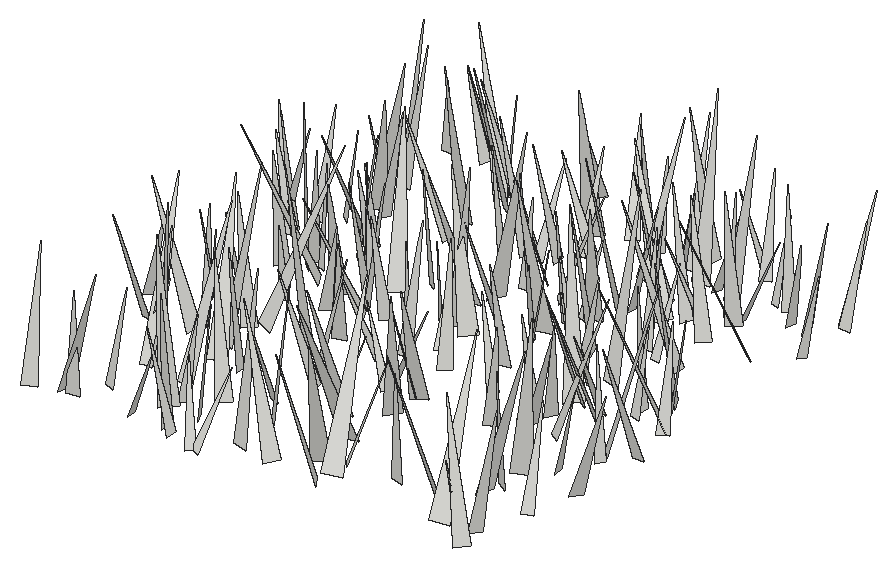
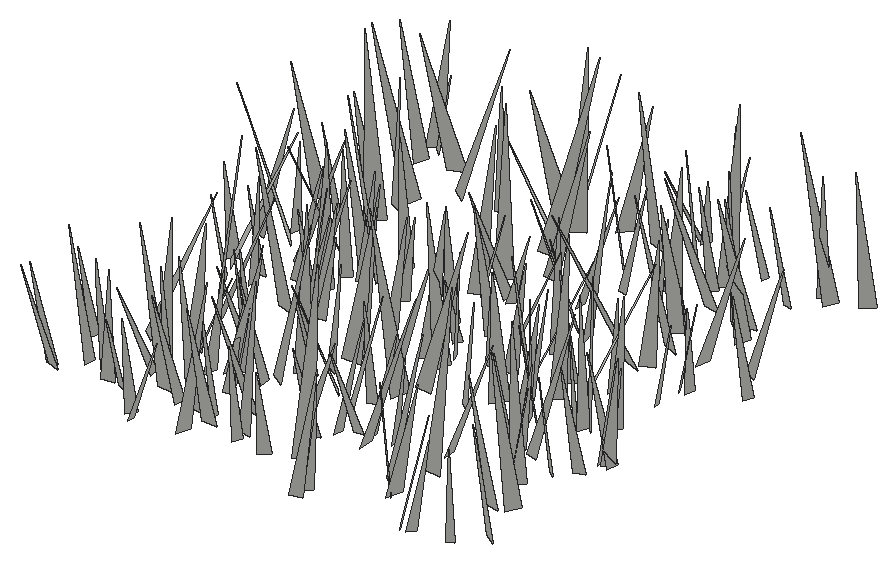
# SketchUp Ruby script. Lengths in inches.
U = 1.inch
M = Sketchup.active_model
def pt(a) = Geom::Point3d.new(a.map { |v| v * U })
def face(e, loops, mat)
  f = e.add_face(loops[0].map { |a| pt(a) })
  loops[1..].each { |l| e.add_face(l.map { |a| pt(a) }).erase! }
  f.material = f.back_material = mat if mat
  f
end
# faces: each face lists its corners as indices into pts; further lists are holes
def faces(e, pts, list, mat = nil) = list.each { |f| face(e, (f[0].is_a?(Array) ? f : [f]).map { |l| l.map { |i| pts[i] } }, mat) }
# xy, xz, yz: faces in a plane at the given z, y or x. An outline is a flat list of corners, or four numbers for a rectangle; further outlines are holes
def ring(l) = l.size == 4 ? [[l[0], l[1]], [l[2], l[1]], [l[2], l[3]], [l[0], l[3]]] : l.each_slice(2).to_a
def flat(e, list, mat, &to3) = list.each { |f| face(e, (f[0].is_a?(Array) ? f : [f]).map { |l| ring(l).map { |u, v| to3.(u, v) } }, mat) }
def xy(e, z, list, mat = nil) = flat(e, list, mat) { |x, y| [x, y, z] }
def xz(e, y, list, mat = nil) = flat(e, list, mat) { |x, z| [x, y, z] }
def yz(e, x, list, mat = nil) = flat(e, list, mat) { |y, z| [x, y, z] }
def lines(e, pts, list) = list.each { |a, b| e.add_line(pt(pts[a]), pt(pts[b])) }
# prism: a flat outline (further loops are holes) pulled along v
def prism(e, loops, v, mat = nil)
  f = face(e, loops, mat); d = Geom::Vector3d.new(v.map { |x| x * U })
  f.pushpull(f.normal.samedirection?(d) ? d.length : -d.length)
end
def box(e, o, s, mat = nil) = prism(e, [[o, [o[0] + s[0], o[1], o[2]], [o[0] + s[0], o[1] + s[1], o[2]], [o[0], o[1] + s[1], o[2]]]], [0, 0, s[2]], mat)
def at(x, y, z, deg = 0) = Geom::Transformation.translation(pt([x, y, z])) * Geom::Transformation.rotation(ORIGIN, Z_AXIS, deg.degrees)
def axes(o, x, y, z) = Geom::Transformation.new([*x, 0, *y, 0, *z, 0, *pt(o).to_a, 1])
def part(name) = M.definitions.add(name)
# library, detail: a bought-in or finely detailed component or shape, given as its bounding box
def library(name, o, s) = part(name).tap { |d| box(d.entities, o, s) }
def detail(e, o, s) = box(e.add_group.entities, o, s)
def put(e, d, t, mat = nil) = e.add_instance(d, t).tap { |i| i.material = mat if mat }
def group(e, t, mat = nil) = e.add_group.tap { |g| g.transformation = t; g.material = mat if mat }.entities
root = M.entities
c1 = part("fur_instance\#9")
p = [[0.8125,0,1.79],[0.67,-0.02,1.48],[0,-0.11,0],[0,0.11,0]]
faces(c1.entities,p,[[0,1,2,3]])
put(root,c1,axes([506.34,202.875,-21.66],[6.83641,-1.96558,0.32372],[-1.94381,-6.83529,-0.45298],[-0.43579,-0.34652,7.09893]))
put(root,c1,axes([507.36,202.43,-21.66],[1.49528,-4.80686,1.53266],[-5.04418,-1.45777,0.34917],[-0.10564,1.56838,5.02194]))
put(root,c1,axes([517.49,202.26,-21.66],[-4.79801,0.15244,1.14259],[0.25589,4.91001,0.4195],[1.12396,-0.46714,4.78206]))
put(root,c1,axes([503.78,201.4375,-21.66],[3.27303,-4.65782,3.06275],[-5.40234,-3.52629,0.41046],[-1.37496,2.76738,5.67799]))
put(root,c1,axes([531.12,203.5,-21.66],[-4.99483,-3.69291,1.05885],[-3.66459,5.10128,0.50484],[1.15306,0.21561,6.19121]))
put(root,c1,axes([520.18,201.25,-21.66],[-3.13044,2.30171,0.23571],[2.28042,3.13636,-0.34054],[0.39127,0.13578,3.8706]))
put(root,c1,axes([512.95,202.91,-21.66],[3.6641,-0.22277,0.06955],[-0.2117,-3.63329,-0.48425],[-0.09821,-0.47926,3.63879]))
put(root,c1,axes([520.61,201.33,-21.66],[0.96645,3.75371,0.08435],[3.72936,-0.9496,-0.47076],[0.43512,-0.19848,3.84744]))
put(root,c1,axes([516.24,203.29,-21.66],[5.75232,0.0292,2.58276],[0.25276,-6.28131,-0.49192],[-2.57052,-0.55229,5.73133]))
put(root,c1,axes([545.98,202.96,-21.66],[-2.17091,-2.72609,1.07786],[-2.90812,2.17161,-0.36485],[0.36901,1.07644,3.46573]))
put(root,c1,axes([546.6,202.58,-21.66],[-4.49758,4.50366,1.60112],[4.72062,4.53017,0.51777],[0.74986,-1.50644,6.34374]))
put(root,c1,axes([529.3,206.34,-21.66],[4.72004,-5.82808,0.22381],[-5.80637,-4.72269,-0.52693],[-0.55017,-0.15829,7.48115]))
put(root,c1,axes([526.38,203.85,-21.66],[-5.76808,3.66085,1.08427],[3.77252,5.76709,0.59739],[0.58783,-1.08949,6.80556]))
put(root,c1,axes([546,204.99,-21.66],[5.31281,-2.73186,1.51927],[-2.91837,-5.40827,0.48055],[-1.11999,1.13346,5.95467]))
put(root,c1,axes([514.47,205.7,-21.66],[-4.81324,5.46383,3.73935],[6.29264,5.21276,0.48307],[2.05886,-3.15867,7.26549]))
put(root,c1,axes([522.86,204.2,-21.66],[2.04699,7.14679,2.15899],[7.40344,-2.23185,0.36858],[-0.96272,-1.9673,7.42502]))
put(root,c1,axes([508.81,205.23,-21.66],[1.57919,4.13225,1.33364],[4.34025,-1.54395,-0.35548],[-0.12772,-1.37428,4.40942]))
put(root,c1,axes([517.51,205.8,-21.66],[4.70905,2.28139,1.77217],[2.5251,-4.89691,-0.40574],[-1.40329,-1.15586,5.21682]))
put(root,c1,axes([540.28,207.46,-21.66],[-3.80657,-5.75041,0.9295],[-5.82495,3.76407,-0.56819],[0.03325,1.08891,6.87272]))
put(root,c1,axes([514.95,206.96,-21.66],[2.82245,-3.27125,1.23973],[-3.47956,-2.78972,0.56063],[-0.36142,1.31172,4.28404]))
put(root,c1,axes([535.97,207.57,-21.66],[-0.76363,-5.08076,1.72351],[-5.30047,0.98391,0.55201],[0.83046,1.60796,5.10809]))
put(root,c1,axes([542.8125,204.45,-21.66],[-2.31741,7.72302,0.72504],[7.71845,2.37113,-0.58682],[0.77216,-0.52327,8.04183]))
put(root,c1,axes([528.875,210.52,-21.66],[0.62863,-8.27068,0.12443],[-8.26435,-0.63324,-0.33804],[-0.34653,0.09834,8.28764]))
put(root,c1,axes([531.41,205.11,-21.66],[-2.88963,7.72101,0.14725],[7.7077,2.8933,-0.45358],[0.4764,0.02131,8.23153]))
put(root,c1,axes([531.25,207.2,-21.66],[3.44436,3.22324,0.28553],[3.18394,-3.45028,0.54084],[-0.57733,0.20181,4.68619]))
put(root,c1,axes([517.37,209.01,-21.66],[-3.57367,4.96866,1.72232],[5.21894,3.60663,0.42422],[0.64547,-1.65218,6.10563]))
put(root,c1,axes([522.4375,208.84,-21.66],[-3.91577,-3.49387,3.17429],[-4.26524,4.38586,-0.43413],[2.02262,2.48468,5.2299]))
put(root,c1,axes([520.36,211.625,-21.66],[-1.29347,-4.18784,0.40951],[-4.17089,1.33267,0.45438],[0.55623,0.25449,4.35943]))
put(root,c1,axes([542.5,210.57,-21.66],[7.35605,-1.97253,1.00478],[-2.03855,-7.39535,0.40615],[-0.86301,0.65556,7.60509]))
put(root,c1,axes([510.33,210.24,-21.66],[4.06784,5.47307,2.7985],[5.78633,-4.54195,0.47187],[-2.07475,-1.93641,6.80288]))
put(root,c1,axes([547.43,209.75,-21.66],[-2.09366,4.25191,0.8072],[4.26644,2.17826,-0.40798],[0.72654,-0.53866,4.72184]))
put(root,c1,axes([509.23,209.8125,-21.66],[1.43263,3.39143,0.32506],[3.34277,-1.46736,0.57677],[-0.65831,-0.07043,3.63615]))
put(root,c1,axes([543.04,212.05,-21.66],[-2.5079,-4.6968,1.95628],[-4.90602,2.8103,0.45782],[1.34828,1.48955,5.3047]))
put(root,c1,axes([526.15,213.41,-21.66],[-0.27695,-6.43694,1.01641],[-6.49492,0.18954,-0.56932],[-0.53231,1.03627,6.4177]))
put(root,c1,axes([508,211.85,-21.66],[5.45486,-2.53583,1.72286],[-2.73109,-5.61705,0.37948],[-1.39279,1.08278,6.00349]))
put(root,c1,axes([513.17,209.35,-21.66],[1.15921,7.66569,0.40932],[7.66684,-1.17697,0.3294],[-0.3873,-0.35503,7.74584]))
put(root,c1,axes([509.18,209.93,-21.66],[-1.39232,7.88876,0.40308],[7.89477,1.37627,0.33483],[-0.26016,-0.45487,8.00369]))
put(root,c1,axes([542.99,214.58,-21.66],[4.39252,-6.51911,2.0007],[-6.79057,-4.39945,0.57342],[-0.62428,1.98542,7.83991]))
put(root,c1,axes([525.11,213.48,-21.66],[2.99336,2.37967,0.42143],[2.41657,-2.95437,-0.48225],[-0.02533,-0.63994,3.79348]))
put(root,c1,axes([529.03,215.77,-21.66],[5.34448,-4.72432,0.68412],[-4.69665,-5.3877,-0.51471],[-0.85369,0.0645,7.11462]))
put(root,c1,axes([515.17,213.81,-21.66],[-5.00491,-0.78513,1.46412],[-0.94309,5.16869,-0.45214],[1.36772,0.69095,5.0459]))
put(root,c1,axes([548.5625,214.52,-21.66],[5.12871,-2.48578,0.55768],[-2.53054,-5.11559,0.47007],[-0.29413,0.66743,5.67995]))
put(root,c1,axes([521.66,215.36,-21.66],[-5.37487,-0.5228,0.79074],[-0.44432,5.41107,0.55741],[0.83736,-0.48456,5.37139]))
put(root,c1,axes([504.14,215.73,-21.66],[-1.82389,-4.57282,0.8897],[-4.65371,1.74485,-0.5721],[-0.21262,1.03617,4.88978]))
put(root,c1,axes([512.76,213.95,-21.66],[-3.64093,6.72533,0.73654],[6.73348,3.68347,-0.34805],[0.65778,-0.48058,7.63972]))
put(root,c1,axes([508.29,216.59,-21.66],[-6.63907,0.80935,0.83748],[0.8673,6.67065,0.42894],[0.7773,-0.53025,6.67446]))
put(root,c1,axes([545,216.74,-21.66],[4.1341,0.32333,0.78637],[0.3951,-4.18703,-0.35553],[-0.75288,-0.42186,4.13146]))
put(root,c1,axes([529.18,218.97,-21.66],[3.47226,-5.91321,0.27335],[-5.89868,-3.48291,-0.41506],[-0.49636,0.02495,6.84473]))
put(root,c1,axes([511.72,216.41,-21.66],[2.95959,7.19025,1.54721],[7.29869,-3.07695,0.338],[-0.90704,-1.29822,7.76818]))
put(root,c1,axes([526.91,217.85,-21.66],[4.6922,-0.3007,0.23761],[-0.32477,-4.66947,0.50417],[-0.20347,0.51889,4.67471]))
put(root,c1,axes([536.24,219.09,-21.66],[2.86346,-4.49186,1.0378],[-4.60706,-2.8331,0.44926],[-0.16992,1.11803,5.30796]))
put(root,c1,axes([501.91,218.77,-21.66],[3.6262,-2.26105,0.60128],[-2.31235,-3.63241,0.28605],[-0.35624,0.56255,4.26378]))
put(root,c1,axes([508.58,217.93,-21.66],[-3.28983,-1.54802,1.9149],[-2.00034,3.5437,-0.57187],[1.43591,1.38997,3.59058]))
put(root,c1,axes([526.23,218.46,-21.66],[-3.21224,1.96871,0.46482],[2.01704,3.18335,0.45637],[0.15311,-0.63315,3.7398]))
put(root,c1,axes([528.625,219.18,-21.66],[-2.84095,-2.72325,0.75235],[-2.80656,2.8428,-0.30791],[0.32453,0.74533,3.9233]))
put(root,c1,axes([517.96,219.02,-21.66],[-7.87878,-1.52664,2.20407],[-1.70967,8.13085,-0.47967],[2.06533,0.90687,8.01097]))
put(root,c1,axes([519.55,218.47,-21.66],[2.50571,3.8301,0.73521],[3.84486,-2.57244,0.29737],[-0.65369,-0.44905,4.56726]))
put(root,c1,axes([511.4,219.66,-21.66],[-3.51075,4.42455,2.16586],[4.8357,3.60279,0.47842],[0.94002,-2.00904,5.62789]))
put(root,c1,axes([538.67,221.18,-21.66],[5.31861,-1.95589,0.12332],[-1.94358,-5.30997,-0.39374],[-0.25139,-0.32717,5.65315]))
put(root,c1,axes([546.67,219.9,-21.66],[-4.5869,1.43943,1.05541],[1.33614,4.69877,-0.60151],[1.18347,0.27406,4.76967]))
put(root,c1,axes([548.74,222.14,-21.66],[-0.82643,-5.48525,0.94931],[-5.54864,0.73423,-0.58792],[-0.44918,1.02229,5.51591]))
put(root,c1,axes([507.12,220.97,-21.66],[-3.57369,-1.9669,1.0397],[-2.0892,3.64317,-0.28897],[0.76478,0.76131,4.06896]))
put(root,c1,axes([518.2,222.53,-21.66],[2.49567,-4.97649,0.70111],[-5.02561,-2.47346,0.33254],[-0.01412,0.77585,5.55727]))
put(root,c1,axes([506.2,220.84,-21.66],[-3.76859,1.24193,1.36163],[1.17189,4.00702,-0.41131],[1.42236,-0.01087,3.94658]))
put(root,c1,axes([522.31,222.1875,-21.66],[-4.25232,-1.15186,0.17503],[-1.13335,4.24309,0.38907],[0.27009,-0.33025,4.38835]))
put(root,c1,axes([536.8125,221.95,-21.66],[7.03431,3.48518,2.0857],[3.73576,-7.18871,-0.58711],[-1.59396,-1.46769,7.82836]))
put(root,c1,axes([538.95,223.29,-21.66],[4.27597,-2.96302,0.67606],[-2.94629,-4.32773,-0.33261],[-0.74558,0.10858,5.19161]))
put(root,c1,axes([537.66,222.88,-21.66],[-3.6167,2.28369,2.19841],[2.80718,3.85669,0.61192],[1.47241,-1.74341,4.23336]))
put(root,c1,axes([543.2,224.2,-21.66],[-2.96525,-5.05492,0.58848],[-5.08807,2.93137,-0.45808],[-0.10025,0.73898,5.84252]))
put(root,c1,axes([546.2,221.31,-21.66],[5.62974,5.25868,1.12192],[5.27805,-5.71471,0.30107],[-1.02693,-0.54292,7.69786]))
put(root,c1,axes([541.26,220.89,-21.66],[3.77289,4.9439,0.17652],[4.9129,-3.7705,0.5956],[-0.58026,0.22179,6.19049]))
put(root,c1,axes([512.39,220.37,-21.66],[3.274,7.7332,0.0389],[7.72076,-3.26624,-0.49451],[0.44025,-0.22856,8.38313]))
put(root,c1,axes([506.95,224.05,-21.66],[-3.35519,-0.75879,1.11745],[-0.66434,3.53232,0.40387],[1.17606,-0.1694,3.41613]))
put(root,c1,axes([533.06,223.35,-21.66],[-3.14224,2.77876,1.0294],[2.91205,3.17344,0.32264],[0.54877,-0.92877,4.18224]))
put(root,c1,axes([510.89,224.71,-21.66],[3.12862,-2.29976,0.97047],[-2.27,-3.26853,-0.42753],[-1.03819,0.21622,3.85932]))
put(root,c1,axes([523.98,223.63,-21.66],[-0.55684,5.82392,2.02647],[6.12632,0.75415,-0.48394],[0.70204,-1.96161,5.83043]))
put(root,c1,axes([541.75,226.18,-21.66],[-0.76321,-4.71965,0.1503],[-4.6984,0.77422,0.45372],[0.47201,0.07524,4.75939]))
put(root,c1,axes([527.8,223.89,-21.66],[3.60386,-3.42869,2.87422],[-4.08632,-4.02533,0.32181],[-1.82182,2.24626,4.96388]))
put(root,c1,axes([514.44,225.5,-21.66],[3.18493,-3.37138,0.77047],[-3.44968,-3.17103,0.3845],[-0.24394,0.82581,4.62191]))
put(root,c1,axes([517.29,226.88,-21.66],[-5.15654,-2.89646,0.02201],[-2.88562,5.14083,0.47427],[0.2514,-0.40276,5.89529]))
put(root,c1,axes([539.73,226.36,-21.66],[-2.91722,-4.26379,0.81225],[-4.33997,2.88016,-0.46811],[0.06569,0.93518,5.14499]))
put(root,c1,axes([547.45,227.24,-21.66],[-5.40162,-4.18627,0.13743],[-4.18531,5.38577,-0.4449],[-0.16419,0.43574,6.81941]))
put(root,c1,axes([513.71,228.14,-21.66],[4.30968,-5.09044,0.61484],[-5.06109,-4.35201,-0.55619],[-0.82219,0.10671,6.64655]))
put(root,c1,axes([519.15,227.27,-21.66],[1.81609,-4.28388,1.69446],[-4.45246,-2.09973,-0.53642],[-1.18256,1.32684,4.62191]))
put(root,c1,axes([531.09,227.37,-21.66],[0.46643,-4.66615,1.44002],[-4.86096,-0.58186,-0.31092],[-0.46655,1.39737,4.67909]))
put(root,c1,axes([525.47,225.99,-21.66],[-2.23531,2.8422,0.49749],[2.78374,2.28983,-0.57415],[0.75919,-0.0278,3.57002]))
put(root,c1,axes([547.81,226.39,-21.66],[-2.87037,3.7349,1.34525],[3.80013,3.06525,-0.40189],[1.14815,-0.80807,4.69329]))
put(root,c1,axes([511.03,228.99,-21.66],[-6.73685,-3.71008,0.0403],[-3.70619,6.73292,0.28887],[0.17463,-0.23362,7.68547]))
put(root,c1,axes([524.21,227.89,-21.66],[-3.74193,-1.93414,1.83822],[-1.95383,4.14237,0.38123],[1.81727,0.47108,4.19495]))
put(root,c1,axes([539.01,226.18,-21.66],[-6.71454,4.39928,1.56364],[4.39375,6.8803,-0.4901],[1.57912,-0.43767,8.0124]))
put(root,c1,axes([544.4,227.19,-21.66],[0.69151,3.97199,1.28395],[4.17346,-0.6309,-0.296],[0.08642,-1.31479,4.02085]))
put(root,c1,axes([521.24,227.43,-21.66],[1.02394,3.35387,1.44831],[3.57422,-1.23084,0.32333],[-0.75567,-1.27715,3.49176]))
put(root,c1,axes([516.77,227.83,-21.66],[3.29579,4.51514,1.8086],[4.80118,-3.36974,-0.33663],[-0.7786,-1.66678,5.57991]))
put(root,c1,axes([538.4,229,-21.66],[-1.63509,-3.83691,0.93062],[-3.94815,1.58786,-0.39017],[-0.00453,1.00909,4.15248]))
put(root,c1,axes([507.09,229.18,-21.66],[4.37094,-3.26497,1.75227],[-3.26747,-4.6741,-0.55863],[-1.74761,0.57306,5.42707]))
put(root,c1,axes([544.18,228.47,-21.66],[-5.10853,0.04095,1.59169],[-0.11644,5.32521,-0.51071],[1.58796,0.52222,5.08311]))
put(root,c1,axes([536.99,229.35,-21.66],[-4.76846,2.17787,1.48985],[2.383,4.8757,0.4998],[1.13316,-1.08876,5.21838]))
put(root,c1,axes([515.02,229.99,-21.66],[4.42222,0.57042,2.59632],[0.96066,-5.04183,-0.52855],[-2.47858,-0.93641,4.42741]))
put(root,c1,axes([536.3,229.85,-21.66],[0.92533,-3.44435,1.34936],[-3.58141,-1.18238,-0.56215],[-0.92618,1.13092,3.52189]))
put(root,c1,axes([525.8125,229.36,-21.66],[-4.89648,5.17695,2.06152],[5.4889,4.95404,0.59637],[0.96057,-1.91907,7.10075]))
put(root,c1,axes([536.8125,229.8,-21.66],[4.06657,-2.17936,1.39694],[-2.40276,-4.14574,0.52683],[-0.9632,1.14071,4.58356]))
put(root,c1,axes([545.53,230.92,-21.66],[-5.52938,-3.456,2.07939],[-3.45701,5.87854,0.57763],[2.07771,0.58365,6.49494]))
put(root,c1,axes([546.32,229.3125,-21.66],[3.3556,2.16226,1.21696],[2.08771,-3.56664,0.58052],[-1.34083,-0.14202,3.94948]))
put(root,c1,axes([523.99,229.91,-21.66],[6.73151,-1.98165,2.55494],[-2.23492,-7.11595,0.36912],[-2.33662,1.09735,7.00742]))
put(root,c1,axes([509,230.79,-21.66],[5.28351,-1.61661,1.62366],[-1.56193,-5.52709,-0.42043],[-1.67632,0.05465,5.50927]))
put(root,c1,axes([508.9375,230.15,-21.66],[4.24793,5.0228,3.04998],[5.34423,-4.86703,0.57187],[-2.44337,-1.91294,6.55335]))
put(root,c1,axes([526.73,232.13,-21.66],[-1.73362,-4.79917,0.85478],[-4.86621,1.65027,-0.60395],[-0.28757,1.00633,5.06683]))
put(root,c1,axes([510,230.55,-21.66],[1.76175,3.91399,1.38102],[4.01071,-1.99148,0.5277],[-1.06803,-1.02224,4.25965]))
put(root,c1,axes([513.99,232.17,-21.66],[1.70929,-4.46495,1.67991],[-4.63149,-1.98085,-0.55231],[-1.1433,1.34907,4.74893]))
put(root,c1,axes([522.8,233.6875,-21.66],[-0.03159,-6.8611,0.78211],[-6.88005,-0.03586,-0.59249],[-0.59273,0.78192,6.83555]))
put(root,c1,axes([513.36,232.03,-21.66],[-4.21315,-2.34987,2.26772],[-2.4638,4.71684,0.31027],[2.14339,0.80291,4.81418]))
put(root,c1,axes([539.45,230.3125,-21.66],[1.82525,7.99707,1.79582],[8.16577,-1.93273,0.30716],[-0.70587,-1.67961,8.19697]))
put(root,c1,axes([530.19,233.59,-21.66],[1.08245,-7.41016,1.80762],[-7.58562,-1.23679,-0.52762],[-0.7977,1.70574,7.47019]))
put(root,c1,axes([529.75,232.49,-21.66],[-4.37552,-5.12362,2.64469],[-5.63456,4.50416,-0.59611],[1.22377,2.41912,6.71129]))
put(root,c1,axes([535.16,233.39,-21.66],[-6.26815,-2.22604,2.13273],[-2.17784,6.6177,0.5065],[2.18193,0.21043,6.63238]))
put(root,c1,axes([516.98,231.4,-21.66],[-5.31707,5.30249,0.96243],[5.27581,5.39738,-0.58989],[1.09932,-0.2564,7.48596]))
put(root,c1,axes([504.62,233.47,-21.66],[-3.50037,2.65675,1.28484],[2.86731,3.53339,0.50538],[0.69832,-1.19104,4.36526]))
put(root,c1,axes([518.54,233.81,-21.66],[2.49829,3.83803,2.30798],[4.11646,-3.0089,0.54773],[-1.76409,-1.58579,4.54664]))
put(root,c1,axes([503.45,234.05,-21.66],[4.85484,-0.93426,0.93937],[-1.01134,-4.91828,0.33525],[-0.85583,0.51221,4.93253]))
put(root,c1,axes([504.66,233.89,-21.66],[-5.03296,-0.41167,1.23228],[-0.52474,5.15421,-0.42127],[1.18855,0.5323,5.03216]))
put(root,c1,axes([509.49,236.74,-21.66],[-2.17037,-5.72704,0.1674],[-5.69455,2.17595,0.61228],[0.63178,-0.0613,6.09382]))
put(root,c1,axes([503.84,234.11,-21.66],[3.17127,-3.30736,3.04126],[-3.82504,-3.9403,-0.2965],[-2.35731,1.94429,4.57249]))
put(root,c1,axes([511.2,233.61,-21.66],[3.52114,3.87417,1.40413],[3.91467,-3.72163,0.45161],[-1.28689,-0.72073,5.21571]))
put(root,c1,axes([542.33,235.3,-21.66],[-7.29173,-1.24054,0.1592],[-1.24954,7.26646,-0.60898],[0.05425,0.6271,7.37139]))
put(root,c1,axes([523.76,235.46,-21.66],[7.67247,-2.21843,2.0813],[-2.41925,-7.8734,0.52613],[-1.84403,1.09916,7.96941]))
put(root,c1,axes([531.95,237.4375,-21.66],[2.97455,-6.14482,0.55918],[-6.16848,-2.94679,0.43089],[0.14598,0.69067,6.8133]))
put(root,c1,axes([530.59,235.63,-21.66],[1.70203,4.17643,2.24286],[4.55719,-2.09788,0.44817],[-1.30578,-1.87783,4.48761]))
put(root,c1,axes([511.05,236.1,-21.66],[0.17752,-3.57602,1.3313],[-3.7929,-0.31113,-0.32997],[-0.41733,1.30655,3.56518]))
put(root,c1,axes([539.82,235.41,-21.66],[0.7,4.04155,0.09862],[4.02713,-0.70587,0.34334],[-0.35517,-0.03822,4.08733]))
put(root,c1,axes([504.86,236.46,-21.66],[-0.99114,4.85366,1.48422],[5.00835,1.18049,-0.51592],[0.82303,-1.33855,4.92689]))
put(root,c1,axes([538.1875,236.34,-21.66],[0.28645,5.00767,1.03913],[5.08565,-0.389,0.47271],[-0.54104,-1.00525,4.99354]))
put(root,c1,axes([531.11,237.04,-21.66],[1.148,3.43718,0.90942],[3.54891,-1.0498,-0.51218],[0.21566,-1.0212,3.58745]))
put(root,c1,axes([524.62,237.9,-21.66],[-0.53957,3.97433,2.02364],[4.38519,0.84425,-0.48882],[0.81275,-1.91664,3.98089]))
put(root,c1,axes([506.53,237.91,-21.66],[2.33806,3.32528,1.40975],[3.5899,-2.32407,-0.47188],[-0.3968,-1.43269,4.03749]))
put(root,c1,axes([545.29,240.36,-21.66],[-4.1792,-5.61615,0.15739],[-5.61189,4.16336,-0.45249],[-0.26934,0.3962,6.98585]))
put(root,c1,axes([532.92,239.52,-21.66],[-3.69542,-5.95234,1.80806],[-6.20183,3.68953,-0.52934],[0.48649,1.82006,6.98615]))
put(root,c1,axes([525.14,240.04,-21.66],[-3.21192,-3.98216,0.77509],[-3.98629,3.28152,0.34045],[0.75355,0.38579,5.10471]))
put(root,c1,axes([536.48,238.92,-21.66],[-2.09497,-3.98677,2.51489],[-4.46346,2.56262,0.34425],[1.51546,2.03632,4.49052]))
put(root,c1,axes([527.8,238.21,-21.66],[3.6626,3.70148,0.35684],[3.71844,-3.64024,-0.40601],[0.03906,-0.53912,5.19141]))
put(root,c1,axes([507.59,240.85,-21.66],[3.73697,-5.4189,0.58942],[-5.45085,-3.71358,0.41766],[0.01126,0.72231,6.56925]))
put(root,c1,axes([514.76,240.49,-21.66],[-5.6933,-0.47947,0.5538],[-0.44449,5.71072,0.37467],[0.58224,-0.32872,5.70116]))
put(root,c1,axes([508.7,240.16,-21.66],[4.80209,-1.99507,1.20954],[-2.10711,-4.89697,0.2883],[-1.00169,0.73669,5.19204]))
put(root,c1,axes([540.88,240.18,-21.66],[3.04965,-4.5466,3.26672],[-5.09549,-3.79519,-0.52522],[-2.31926,2.35973,5.44941]))
put(root,c1,axes([507.76,241.83,-21.66],[-3.40624,-2.616,1.08161],[-2.59295,3.56228,0.44999],[1.13575,0.28715,4.27123]))
put(root,c1,axes([539.54,241.96,-21.66],[-4.06839,-1.50308,0.30492],[-1.46625,4.06536,0.47647],[0.44983,-0.34301,4.31092]))
put(root,c1,axes([533.375,240.54,-21.66],[4.7353,0.6555,1.15241],[0.55235,-4.8611,0.49538],[-1.20525,0.34759,4.75472]))
put(root,c1,axes([534.81,242.5,-21.66],[-5.38028,-3.08502,1.66928],[-3.07413,5.61908,0.47644],[1.68926,0.39986,6.18367]))
put(root,c1,axes([519.33,241.64,-21.66],[-4.34694,-0.07841,1.0456],[-0.20123,4.43859,-0.5037],[1.02905,0.53671,4.31837]))
put(root,c1,axes([536.25,240.79,-21.66],[-6.04879,4.39479,0.23194],[4.40071,6.03643,0.38865],[-0.04117,-0.45072,7.46666]))
put(root,c1,axes([513.92,243.67,-21.66],[-1.04012,-7.65192,1.88155],[-7.84849,1.17518,0.4406],[0.70237,1.80029,7.70971]))
put(root,c1,axes([534.6,243.67,-21.66],[1.52104,-3.59534,0.18519],[-3.58042,-1.53172,-0.32978],[-0.37596,0.04131,3.88989]))
put(root,c1,axes([523.81,243.1875,-21.66],[-5.16901,0.01394,1.37798],[0.15537,5.32107,0.52899],[1.36927,-0.55116,5.14189]))
put(root,c1,axes([537.81,241.9,-21.66],[-5.43325,1.77797,0.85582],[1.73658,5.49897,-0.39929],[0.93695,0.1182,5.7028]))
put(root,c1,axes([521.25,242.22,-21.66],[-5.82181,0.2065,0.70872],[0.14567,5.84473,-0.50632],[0.72368,0.48471,5.80343]))
put(root,c1,axes([520.95,243.35,-21.66],[-7.49054,-0.65717,0.9559],[-0.61994,7.54719,0.33069],[0.98046,-0.24861,7.51203]))
put(root,c1,axes([541.17,243.64,-21.66],[-3.30956,4.62511,3.28339],[5.43338,3.67626,0.29816],[1.62808,-2.86687,5.67942]))
put(root,c1,axes([548.55,243.02,-21.66],[3.49135,-1.63355,1.08284],[-1.80913,-3.53699,0.49727],[-0.7537,0.9229,3.8224]))
put(root,c1,axes([505.3,244.25,-21.66],[5.59181,-3.37862,1.09906],[-3.46581,-5.63815,0.30113],[-0.78177,0.82912,6.52631]))
put(root,c1,axes([522.52,242.19,-21.66],[-0.04754,4.40868,0.34675],[4.41199,0.07095,-0.29716],[0.30179,-0.34273,4.39891]))
put(root,c1,axes([525.99,244.9,-21.66],[-4.59292,1.38597,0.57425],[1.45174,4.5724,0.57548],[0.37836,-0.71958,4.76284]))
put(root,c1,axes([540.14,244.29,-21.66],[0.9151,5.15761,1.58711],[5.35443,-1.06795,0.38322],[-0.67079,-1.48856,5.22413]))
put(root,c1,axes([541.2,244.74,-21.66],[3.9948,0.59542,0.26899],[0.55235,-3.96784,0.58004],[-0.34899,0.53573,3.99706]))
put(root,c1,axes([544.66,246.52,-21.66],[4.24921,-1.39082,0.67887],[-1.35455,-4.30166,-0.33452],[-0.74864,-0.11098,4.4585]))
put(root,c1,axes([506.81,245.02,-21.66],[1.78136,5.8506,1.71123],[6.09225,-1.76893,-0.29408],[-0.20572,-1.72409,6.10871]))
put(root,c1,axes([515.69,246.88,-21.66],[-3.47477,-5.64058,1.59223],[-5.83486,3.50381,-0.32112],[0.55295,1.52727,6.61718]))
put(root,c1,axes([546.27,246.5625,-21.66],[5.73568,-0.06882,1.05766],[0.01363,-5.81521,-0.45231],[-1.05981,-0.44725,5.71823]))
put(root,c1,axes([524.84,244.93,-21.66],[-1.136,4.49998,0.83575],[4.53043,1.22799,-0.4539],[0.65076,-0.69355,4.61891]))
put(root,c1,axes([523.41,248.13,-21.66],[4.47344,-6.57845,1.38646],[-6.62258,-4.59864,-0.45163],[-1.15746,0.88686,7.94253]))
put(root,c1,axes([538.85,246.25,-21.66],[1.36969,7.27883,2.41401],[7.66649,-1.2409,-0.6083],[0.18385,-2.48268,7.38156]))
put(root,c1,axes([533.01,247.28,-21.66],[4.24569,0.44069,0.96407],[0.53821,-4.32495,-0.39327],[-0.91322,-0.50013,4.25034]))
put(root,c1,axes([529.52,247.97,-21.66],[1.75829,5.41715,3.42251],[6.36736,-1.87488,-0.30363],[-0.71818,-3.36006,5.68726]))
put(root,c1,axes([536.61,247.22,-21.66],[4.56446,-0.76979,0.5853],[-0.81155,-4.58493,0.29877],[-0.52586,0.39409,4.61927]))
put(root,c1,axes([530.97,244.99,-21.66],[1.53253,6.73152,0.42824],[6.72346,-1.5597,0.45586],[-0.5402,-0.31526,6.8887]))
put(root,c1,axes([514.34,248.5,-21.66],[3.53151,3.08583,1.68165],[3.37882,-3.63698,-0.42174],[-0.96639,-1.43941,4.67077]))
put(root,c1,axes([543.22,248.08,-21.66],[-1.15441,5.11883,1.74969],[5.40957,1.09949,0.35248],[0.0216,-1.78472,5.23554]))
put(root,c1,axes([534.83,247.39,-21.66],[-0.16365,8.04006,1.71484],[8.20749,0.06185,0.49328],[-0.46944,-1.72152,8.02659]))
put(root,c1,axes([541.65,248.23,-21.66],[1.21689,3.56799,0.58582],[3.55761,-1.29191,0.47847],[-0.64586,-0.39367,3.73931]))
put(root,c1,axes([548.37,248.6,-21.66],[0.17579,4.7582,1.26729],[4.89735,-0.03702,-0.54033],[0.51227,-1.27889,4.73069]))
put(root,c1,axes([529.3,249.0625,-21.66],[-3.40994,2.09099,1.78678],[2.1335,3.80705,-0.3836],[1.73581,-0.57158,3.98156]))
put(root,c1,axes([514.11,248.3,-21.66],[-6.63605,2.7216,0.19643],[2.70208,6.62626,-0.52374],[0.38006,0.41041,7.15332]))
put(root,c1,axes([503.76,249.12,-21.66],[2.58353,5.00263,1.49189],[5.09313,-2.78069,0.50442],[-1.14546,-1.08079,5.60772]))
put(root,c1,axes([533.54,250.61,-21.66],[-6.59669,1.20746,2.1658],[1.44471,6.87425,0.5679],[2.0153,-0.97558,6.6822]))
put(root,c1,axes([532.63,248.46,-21.66],[-0.26987,6.47949,0.83868],[6.52839,0.23411,0.29205],[-0.25936,-0.84936,6.47853]))
put(root,c1,axes([505.91,251.42,-21.66],[0.58274,-3.68979,0.92218],[-3.78198,-0.46356,0.53511],[0.40205,0.98748,3.697]))
put(root,c1,axes([548.03,248.9,-21.66],[1.54833,5.59255,0.52827],[5.59137,-1.58705,0.41342],[-0.54067,-0.39706,5.78818]))
put(root,c1,axes([510.51,251.98,-21.66],[-3.88391,-3.01754,1.00768],[-2.99103,4.00531,0.46572],[1.08383,0.24005,4.89626]))
put(root,c1,axes([526.26,249.5,-21.66],[-3.1637,4.01487,0.30871],[3.99884,3.17867,-0.35895],[0.47305,-0.01931,5.09895]))
put(root,c1,axes([520.04,253.33,-21.66],[2.51881,-4.55482,0.15905],[-4.51842,-2.51942,-0.59372],[-0.59628,-0.14918,5.17091]))
put(root,c1,axes([537.94,251.76,-21.66],[-3.79704,-0.30553,0.54536],[-0.26679,3.82814,0.28712],[0.56533,-0.2455,3.79848]))
put(root,c1,axes([519.86,251.88,-21.66],[-3.10303,1.40825,1.48641],[1.65077,3.31728,0.3033],[1.21143,-0.91317,3.39411]))
put(root,c1,axes([509.41,251.95,-21.66],[-3.58724,1.8714,1.40372],[2.1412,3.66165,0.59026],[0.94225,-1.19623,4.00275]))
put(root,c1,axes([538.57,250.88,-21.66],[-3.00951,3.51493,1.30262],[3.55292,3.20728,-0.44587],[1.1951,-0.68362,4.60577]))
